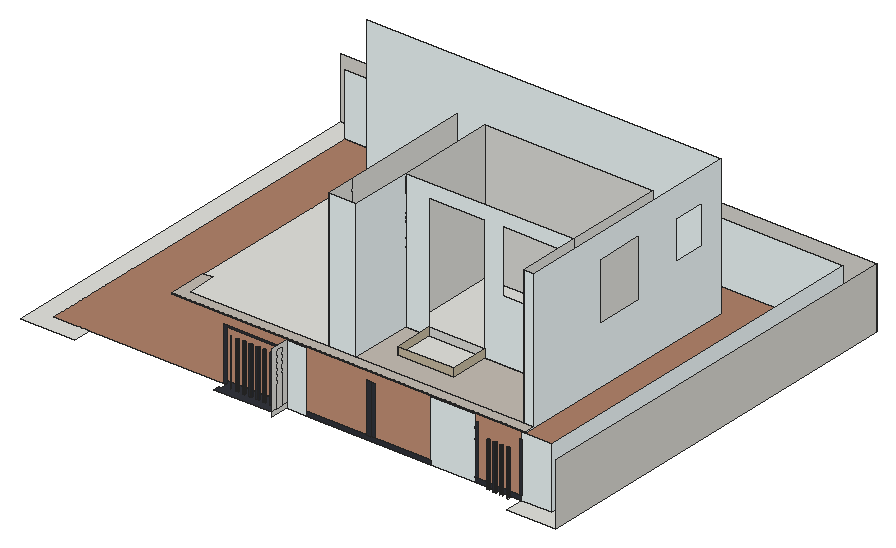
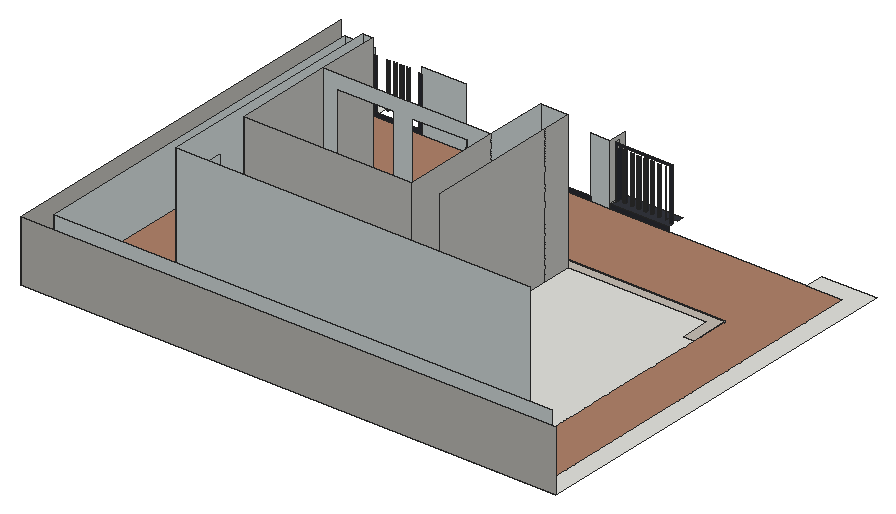
# SketchUp Ruby script. Lengths in inches.
U = 1.inch
M = Sketchup.active_model
def pt(a) = Geom::Point3d.new(a.map { |v| v * U })
def face(e, loops, mat)
  f = e.add_face(loops[0].map { |a| pt(a) })
  loops[1..].each { |l| e.add_face(l.map { |a| pt(a) }).erase! }
  f.material = f.back_material = mat if mat
  f
end
# faces: each face lists its corners as indices into pts; further lists are holes
def faces(e, pts, list, mat = nil) = list.each { |f| face(e, (f[0].is_a?(Array) ? f : [f]).map { |l| l.map { |i| pts[i] } }, mat) }
# xy, xz, yz: faces in a plane at the given z, y or x. An outline is a flat list of corners, or four numbers for a rectangle; further outlines are holes
def ring(l) = l.size == 4 ? [[l[0], l[1]], [l[2], l[1]], [l[2], l[3]], [l[0], l[3]]] : l.each_slice(2).to_a
def flat(e, list, mat, &to3) = list.each { |f| face(e, (f[0].is_a?(Array) ? f : [f]).map { |l| ring(l).map { |u, v| to3.(u, v) } }, mat) }
def xy(e, z, list, mat = nil) = flat(e, list, mat) { |x, y| [x, y, z] }
def xz(e, y, list, mat = nil) = flat(e, list, mat) { |x, z| [x, y, z] }
def yz(e, x, list, mat = nil) = flat(e, list, mat) { |y, z| [x, y, z] }
def lines(e, pts, list) = list.each { |a, b| e.add_line(pt(pts[a]), pt(pts[b])) }
# prism: a flat outline (further loops are holes) pulled along v
def prism(e, loops, v, mat = nil)
  f = face(e, loops, mat); d = Geom::Vector3d.new(v.map { |x| x * U })
  f.pushpull(f.normal.samedirection?(d) ? d.length : -d.length)
end
def box(e, o, s, mat = nil) = prism(e, [[o, [o[0] + s[0], o[1], o[2]], [o[0] + s[0], o[1] + s[1], o[2]], [o[0], o[1] + s[1], o[2]]]], [0, 0, s[2]], mat)
def at(x, y, z, deg = 0) = Geom::Transformation.translation(pt([x, y, z])) * Geom::Transformation.rotation(ORIGIN, Z_AXIS, deg.degrees)
def axes(o, x, y, z) = Geom::Transformation.new([*x, 0, *y, 0, *z, 0, *pt(o).to_a, 1])
def part(name) = M.definitions.add(name)
# library, detail: a bought-in or finely detailed component or shape, given as its bounding box
def library(name, o, s) = part(name).tap { |d| box(d.entities, o, s) }
def detail(e, o, s) = box(e.add_group.entities, o, s)
def put(e, d, t, mat = nil) = e.add_instance(d, t).tap { |i| i.material = mat if mat }
def group(e, t, mat = nil) = e.add_group.tap { |g| g.transformation = t; g.material = mat if mat }.entities
root = M.entities
M.materials.add("[Concrete Tile]").color = [203, 190, 164]
M.materials.add("[Field Rectangle Tile]").color = [196, 189, 179]
M.materials.add("[Formica Laminate Dark]1").color = [50, 53, 60]
M.materials.add("[Pavers Driveway Brick]").color = [176, 130, 106]
M.materials.add("[Terrazzo Tile Light]").color = [219, 217, 210]
M.materials.add("[White Subway Tile]").color = [243, 252, 253]
M.materials.add("[White Subway Tile]1").color = [243, 252, 253]
xy(root,0,[[0,0,0,2816.0625,3762.625,2816.0625,3762.625,0,3421.78,0,3421.78,129.42,3633.2,129.42,3633.2,2686.64,129.42,2686.64,129.42,129.42,383.65,129.42,383.65,0],[477.43,733.79,2968.68,2442.87]])
xy(root,0,[[[129.42,129.42,3633.2,2686.64],[477.43,733.79,2968.68,2442.87]]],"[Pavers Driveway Brick]")
xy(root,9,[[1882.4375,963.83,2273.5625,1239.01],[1717.43,1239.01,2898.76,1933.89]])
xy(root,9,[[477.43,733.79,2968.68,733.79,2968.68,803.71,547.35,803.71,547.35,1008.89,477.43,1008.89],[1717.43,803.71,2898.76,803.71,2898.76,1239.01,2273.5625,1239.01,2273.5625,963.83,1882.4375,963.83,1882.4375,1239.01,1717.43,1239.01]],"[Field Rectangle Tile]")
xy(root,29.875,[[3376.3,55.58,3373.8,55.72,3371.41,56.51,3369.31,57.89,3367.64,59.76,3366.51,62.01,3365.99,64.47,3366.14,66.98,3366.92,69.36,3368.3,71.46,3370.18,73.14,3372.42,74.27,3374.88,74.78,3377.39,74.64,3379.77,73.85,3381.875,72.47,3383.55,70.6,3384.68,68.35,3385.19,65.89,3385.05,63.38,3384.26,61,3382.88,58.9,3381.01,57.22,3378.76,56.09]])
xy(root,29.875,[[[1357.59,0,1765.91,0,1765.91,44.85,1752.89,44.85,1752.89,92.78,1765.91,92.78,1765.91,129.42,1357.59,129.42,1357.59,92.78,1376.86,92.78,1376.86,44.85,1357.59,44.85],[1663.87,55.58,1661.36,55.72,1658.97,56.51,1656.87,57.89,1655.2,59.76,1654.07,62.01,1653.56,64.47,1653.7,66.98,1654.49,69.36,1655.86,71.46,1657.74,73.14,1659.98,74.27,1662.44,74.78,1664.95,74.64,1667.34,73.85,1669.4375,72.47,1671.11,70.6,1672.24,68.35,1672.75,65.89,1672.61,63.38,1671.82,61,1670.45,58.9,1668.57,57.22,1666.33,56.09],[1417.24,55.58,1414.73,55.72,1412.35,56.51,1410.25,57.89,1408.57,59.76,1407.44,62.01,1406.93,64.47,1407.07,66.98,1407.86,69.36,1409.24,71.46,1411.11,73.14,1413.36,74.27,1415.82,74.78,1418.33,74.64,1420.71,73.85,1422.8125,72.47,1424.49,70.6,1425.62,68.35,1426.13,65.89,1425.99,63.38,1425.2,61,1423.82,58.9,1421.95,57.22,1419.7,56.09],[1616.43,55.58,1613.92,55.72,1611.54,56.51,1609.43,57.89,1607.76,59.76,1606.63,62.01,1606.12,64.47,1606.26,66.98,1607.05,69.36,1608.43,71.46,1610.3,73.14,1612.54,74.27,1615,74.78,1617.51,74.64,1619.9,73.85,1622,72.47,1623.67,70.6,1624.8,68.35,1625.32,65.89,1625.17,63.38,1624.39,61,1623.01,58.9,1621.13,57.22,1618.89,56.09],[1472.87,55.58,1470.36,55.72,1467.97,56.51,1465.87,57.89,1464.2,59.76,1463.07,62.01,1462.56,64.47,1462.7,66.98,1463.49,69.36,1464.86,71.46,1466.74,73.14,1468.98,74.27,1471.44,74.78,1473.95,74.64,1476.34,73.85,1478.4375,72.47,1480.11,70.6,1481.24,68.35,1481.75,65.89,1481.61,63.38,1480.82,61,1479.45,58.9,1477.57,57.22,1475.33,56.09],[1518.99,55.58,1516.48,55.72,1514.1,56.51,1512,57.89,1510.32,59.76,1509.19,62.01,1508.68,64.47,1508.82,66.98,1509.61,69.36,1510.99,71.46,1512.86,73.14,1515.11,74.27,1517.57,74.78,1520.08,74.64,1522.46,73.85,1524.5625,72.47,1526.24,70.6,1527.37,68.35,1527.88,65.89,1527.74,63.38,1526.95,61,1525.57,58.9,1523.7,57.22,1521.45,56.09],[1714.37,55.58,1711.86,55.72,1709.47,56.51,1707.37,57.89,1705.7,59.76,1704.57,62.01,1704.06,64.47,1704.2,66.98,1704.99,69.36,1706.36,71.46,1708.24,73.14,1710.48,74.27,1712.94,74.78,1715.45,74.64,1717.84,73.85,1719.9375,72.47,1721.61,70.6,1722.74,68.35,1723.25,65.89,1723.11,63.38,1722.32,61,1720.95,58.9,1719.07,57.22,1716.83,56.09],[1566.87,55.58,1564.36,55.72,1561.97,56.51,1559.87,57.89,1558.2,59.76,1557.07,62.01,1556.56,64.47,1556.7,66.98,1557.49,69.36,1558.86,71.46,1560.74,73.14,1562.98,74.27,1565.44,74.78,1567.95,74.64,1570.34,73.85,1572.4375,72.47,1574.11,70.6,1575.24,68.35,1575.75,65.89,1575.61,63.38,1574.82,61,1573.45,58.9,1571.57,57.22,1569.33,56.09]]],"[Formica Laminate Dark]1")
xz(root,92.78,[[1357.59,29.875,1357.59,402.23,1765.91,402.23,1765.91,29.875,1752.89,29.875,1752.89,387.92,1376.86,387.92,1376.86,29.875]],"[Formica Laminate Dark]1")
xz(root,129.42,[[1357.59,0,1765.91,29.875],[1905.75,0,2778.47,29.875],[3092.67,0,3421.78,29.875],[2330.84,29.875,2358.7,373.47],[2358.7,29.875,2386.55,373.47],
  [3092.67,29.875,3111.49,384.04],[3407.39,29.875,3421.78,384.04]],"[Formica Laminate Dark]1")
xz(root,129.42,[[1765.91,0,1905.75,429.3125],[2778.47,0,3092.67,429.3125],[3421.78,0,3633.2,429.3125]],"[White Subway Tile]1")
xz(root,733.79,[[477.43,0,2968.68,9]])
xz(root,803.71,[[1522.59,9,1717.43,973.375],[2898.76,9,2968.68,973.375]],"[White Subway Tile]")
xz(root,963.83,[[1882.4375,9,2273.5625,62.21]],"[Concrete Tile]")
xz(root,1239.01,[[1882.4375,9,2273.5625,62.21]])
xz(root,1239.01,[[[1717.43,9,1882.4375,9,1882.4375,877.21,2273.5625,877.21,2273.5625,9,2898.76,9,2898.76,973.375,1717.43,973.375],[2398.08,439.46,2800.45,879.09]]],"[White Subway Tile]")
xz(root,1933.89,[[1717.43,9,2898.76,973.375]])
xz(root,2442.87,[[477.43,0,2968.68,973.375]],"[White Subway Tile]")
xz(root,2686.64,[[129.42,0,3633.2,429.3125]],"[White Subway Tile]1")
xz(root,2816.0625,[[0,0,3762.625,429.3125]],"[Terrazzo Tile Light]")
yz(root,1522.59,[[803.71,9,1008.89,973.375],[1008.89,9,1933.89,973.375]])
yz(root,1717.43,[[1239.01,9,1933.89,973.375]])
yz(root,1717.43,[[803.71,9,1239.01,973.375]],"[White Subway Tile]")
yz(root,1752.89,[[44.85,29.875,92.78,357.02]],"[Formica Laminate Dark]1")
yz(root,1765.91,[[0,0,129.42,29.875],[0,29.875,0,429.3125,129.42,429.3125,129.42,29.875,92.78,29.875,92.78,402.23,44.85,402.23,44.85,29.875],[44.85,29.875,92.78,402.23]])
yz(root,1882.4375,[[963.83,9,1239.01,62.21]],"[Concrete Tile]")
yz(root,2273.5625,[[963.83,9,1239.01,62.21]],"[Concrete Tile]")
yz(root,2898.76,[[803.71,9,1239.01,973.375],[1239.01,9,1933.89,973.375]])
yz(root,2968.68,[[[733.79,0,2442.87,0,2442.87,973.375,803.71,973.375,803.71,9,733.79,9],[1375.57,402.84,1724.7,809.34],[2046.63,498.46,2278.38,771.33]]],"[White Subway Tile]")
yz(root,3633.2,[[129.42,0,2686.64,429.3125]],"[White Subway Tile]1")
yz(root,3762.625,[[0,0,2816.0625,429.3125]],"[Terrazzo Tile Light]")
p = [[1462.7,66.98,29.875],[1462.56,64.47,29.875],[1462.56,64.47,357.02],[1462.7,66.98,357.02],[1508.82,66.98,29.875],[1508.68,64.47,29.875],
  [1508.68,64.47,357.02],[1508.82,66.98,357.02],[1556.7,66.98,29.875],[1556.56,64.47,29.875],[1556.56,64.47,357.02],[1556.7,66.98,357.02],
  [1606.26,66.98,29.875],[1606.12,64.47,29.875],[1606.12,64.47,357.02],[1606.26,66.98,357.02],[1653.7,66.98,29.875],[1653.56,64.47,29.875],
  [1653.56,64.47,357.02],[1653.7,66.98,357.02],[1704.2,66.98,29.875],[1704.06,64.47,29.875],[1704.06,64.47,357.02],[1704.2,66.98,357.02],
  [3226.76,66.98,29.875],[3226.62,64.47,29.875],[3226.62,64.47,342.54],[3226.76,66.98,342.54],[3272.39,66.98,29.875],[3272.24,64.47,29.875],
  [3272.24,64.47,342.54],[3272.39,66.98,342.54],[3318.51,66.98,29.875],[3318.37,64.47,29.875],[3318.37,64.47,342.54],[3318.51,66.98,342.54],
  [3366.14,66.98,29.875],[3365.99,64.47,29.875],[3365.99,64.47,342.54],[3366.14,66.98,342.54],[1426.13,65.89,29.875],[1425.62,68.35,29.875],
  [1425.62,68.35,357.02],[1426.13,65.89,357.02],[1481.75,65.89,29.875],[1481.24,68.35,29.875],[1481.24,68.35,357.02],[1481.75,65.89,357.02],
  [1527.88,65.89,29.875],[1527.37,68.35,29.875],[1527.37,68.35,357.02],[1527.88,65.89,357.02],[1575.75,65.89,29.875],[1575.24,68.35,29.875],
  [1575.24,68.35,357.02],[1575.75,65.89,357.02],[1625.32,65.89,29.875],[1624.8,68.35,29.875],[1624.8,68.35,357.02],[1625.32,65.89,357.02],
  [1672.75,65.89,29.875],[1672.24,68.35,29.875],[1672.24,68.35,357.02],[1672.75,65.89,357.02],[1723.25,65.89,29.875],[1722.74,68.35,29.875],
  [1722.74,68.35,357.02],[1723.25,65.89,357.02],[3245.82,65.89,29.875],[3245.3,68.35,29.875],[3245.3,68.35,342.54],[3245.82,65.89,342.54],
  [3291.44,65.89,29.875],[3290.93,68.35,29.875],[3290.93,68.35,342.54],[3291.44,65.89,342.54],[3337.57,65.89,29.875],[3337.05,68.35,29.875],
  [3337.05,68.35,342.54],[3337.57,65.89,342.54],[3385.19,65.89,29.875],[3384.68,68.35,29.875],[3384.68,68.35,342.54],[3385.19,65.89,342.54],
  [1463.49,69.36,29.875],[1463.49,69.36,357.02],[1509.61,69.36,29.875],[1509.61,69.36,357.02],[1557.49,69.36,29.875],[1557.49,69.36,357.02],
  [1607.05,69.36,29.875],[1607.05,69.36,357.02],[1654.49,69.36,29.875],[1654.49,69.36,357.02],[1704.99,69.36,29.875],[1704.99,69.36,357.02],
  [3227.55,69.36,29.875],[3227.55,69.36,342.54],[3273.17,69.36,29.875],[3273.17,69.36,342.54],[3319.3,69.36,29.875],[3319.3,69.36,342.54],
  [3366.92,69.36,29.875],[3366.92,69.36,342.54],[1424.49,70.6,29.875],[1424.49,70.6,357.02],[1480.11,70.6,29.875],[1480.11,70.6,357.02],
  [1526.24,70.6,29.875],[1526.24,70.6,357.02],[1574.11,70.6,29.875],[1574.11,70.6,357.02],[1623.67,70.6,29.875],[1623.67,70.6,357.02],
  [1671.11,70.6,29.875],[1671.11,70.6,357.02],[1721.61,70.6,29.875],[1721.61,70.6,357.02],[3244.17,70.6,29.875],[3244.17,70.6,342.54],
  [3289.8,70.6,29.875],[3289.8,70.6,342.54],[3335.92,70.6,29.875],[3335.92,70.6,342.54],[3383.55,70.6,29.875],[3383.55,70.6,342.54],
  [1464.86,71.46,29.875],[1464.86,71.46,357.02],[1510.99,71.46,29.875],[1510.99,71.46,357.02],[1558.86,71.46,29.875],[1558.86,71.46,357.02],
  [1608.43,71.46,29.875],[1608.43,71.46,357.02],[1655.86,71.46,29.875],[1655.86,71.46,357.02],[1706.36,71.46,29.875],[1706.36,71.46,357.02],
  [3228.93,71.46,29.875],[3228.93,71.46,342.54],[3274.55,71.46,29.875],[3274.55,71.46,342.54],[3320.68,71.46,29.875],[3320.68,71.46,342.54],
  [3368.3,71.46,29.875],[3368.3,71.46,342.54],[1422.8125,72.47,29.875],[1422.8125,72.47,357.02],[1478.4375,72.47,29.875],[1478.4375,72.47,357.02],
  [1524.5625,72.47,29.875],[1524.5625,72.47,357.02],[1572.4375,72.47,29.875],[1572.4375,72.47,357.02],[1622,72.47,29.875],[1622,72.47,357.02],
  [1669.4375,72.47,29.875],[1669.4375,72.47,357.02],[1719.9375,72.47,29.875],[1719.9375,72.47,357.02],[3242.5,72.47,29.875],[3242.5,72.47,342.54],
  [3288.125,72.47,29.875],[3288.125,72.47,342.54],[3334.25,72.47,29.875],[3334.25,72.47,342.54],[3381.875,72.47,29.875],[3381.875,72.47,342.54],
  [1466.74,73.14,29.875],[1466.74,73.14,357.02],[1512.86,73.14,29.875],[1512.86,73.14,357.02],[1560.74,73.14,29.875],[1560.74,73.14,357.02],
  [1610.3,73.14,29.875],[1610.3,73.14,357.02],[1657.74,73.14,29.875],[1657.74,73.14,357.02],[1708.24,73.14,29.875],[1708.24,73.14,357.02],
  [3230.8,73.14,29.875],[3230.8,73.14,342.54],[3276.43,73.14,29.875],[3276.43,73.14,342.54],[3322.55,73.14,29.875],[3322.55,73.14,342.54],
  [3370.18,73.14,29.875],[3370.18,73.14,342.54],[1420.71,73.85,29.875],[1420.71,73.85,357.02],[1476.34,73.85,29.875],[1476.34,73.85,357.02],
  [1522.46,73.85,29.875],[1522.46,73.85,357.02],[1570.34,73.85,29.875],[1570.34,73.85,357.02],[1619.9,73.85,29.875],[1619.9,73.85,357.02],
  [1667.34,73.85,29.875],[1667.34,73.85,357.02],[1717.84,73.85,29.875],[1717.84,73.85,357.02],[3240.4,73.85,29.875],[3240.4,73.85,342.54],
  [3286.02,73.85,29.875],[3286.02,73.85,342.54],[3332.15,73.85,29.875],[3332.15,73.85,342.54],[3379.77,73.85,29.875],[3379.77,73.85,342.54],
  [1468.98,74.27,29.875],[1468.98,74.27,357.02],[1515.11,74.27,29.875],[1515.11,74.27,357.02],[1562.98,74.27,29.875],[1562.98,74.27,357.02],
  [1612.54,74.27,29.875],[1612.54,74.27,357.02],[1659.98,74.27,29.875],[1659.98,74.27,357.02],[1710.48,74.27,29.875],[1710.48,74.27,357.02],
  [3233.04,74.27,29.875],[3233.04,74.27,342.54],[3278.67,74.27,29.875],[3278.67,74.27,342.54],[3324.79,74.27,29.875],[3324.79,74.27,342.54],
  [3372.42,74.27,29.875],[3372.42,74.27,342.54],[1418.33,74.64,29.875],[1418.33,74.64,357.02],[1473.95,74.64,29.875],[1473.95,74.64,357.02],
  [1520.08,74.64,29.875],[1520.08,74.64,357.02],[1567.95,74.64,29.875],[1567.95,74.64,357.02],[1617.51,74.64,29.875],[1617.51,74.64,357.02],
  [1664.95,74.64,29.875],[1664.95,74.64,357.02],[1715.45,74.64,29.875],[1715.45,74.64,357.02],[3238.01,74.64,29.875],[3238.01,74.64,342.54],
  [3283.64,74.64,29.875],[3283.64,74.64,342.54],[3329.76,74.64,29.875],[3329.76,74.64,342.54],[3377.39,74.64,29.875],[3377.39,74.64,342.54],
  [1471.44,74.78,29.875],[1471.44,74.78,357.02],[1517.57,74.78,29.875],[1517.57,74.78,357.02],[1565.44,74.78,29.875],[1565.44,74.78,357.02],
  [1615,74.78,29.875],[1615,74.78,357.02],[1662.44,74.78,29.875],[1662.44,74.78,357.02],[1712.94,74.78,29.875],[1712.94,74.78,357.02],
  [3235.5,74.78,29.875],[3235.5,74.78,342.54],[3281.13,74.78,29.875],[3281.13,74.78,342.54],[3327.25,74.78,29.875],[3327.25,74.78,342.54],
  [3374.88,74.78,29.875],[3374.88,74.78,342.54]]
faces(root,p,[[0,1,2,3],[4,5,6,7],[8,9,10,11],[12,13,14,15],[16,17,18,19],[20,21,22,23],[24,25,26,27],[28,29,30,31],
  [32,33,34,35],[36,37,38,39],[40,41,42,43],[44,45,46,47],[48,49,50,51],[52,53,54,55],[56,57,58,59],[60,61,62,63],
  [64,65,66,67],[68,69,70,71],[72,73,74,75],[76,77,78,79],[80,81,82,83],[84,0,3,85],[86,4,7,87],[88,8,11,89],
  [90,12,15,91],[92,16,19,93],[94,20,23,95],[96,24,27,97],[98,28,31,99],[100,32,35,101],[102,36,39,103],[41,104,105,42],
  [45,106,107,46],[49,108,109,50],[53,110,111,54],[57,112,113,58],[61,114,115,62],[65,116,117,66],[69,118,119,70],[73,120,121,74],
  [77,122,123,78],[81,124,125,82],[126,84,85,127],[128,86,87,129],[130,88,89,131],[132,90,91,133],[134,92,93,135],[136,94,95,137],
  [138,96,97,139],[140,98,99,141],[142,100,101,143],[144,102,103,145],[104,146,147,105],[106,148,149,107],[108,150,151,109],[110,152,153,111],
  [112,154,155,113],[114,156,157,115],[116,158,159,117],[118,160,161,119],[120,162,163,121],[122,164,165,123],[124,166,167,125],[168,126,127,169],
  [170,128,129,171],[172,130,131,173],[174,132,133,175],[176,134,135,177],[178,136,137,179],[180,138,139,181],[182,140,141,183],[184,142,143,185],
  [186,144,145,187],[146,188,189,147],[148,190,191,149],[150,192,193,151],[152,194,195,153],[154,196,197,155],[156,198,199,157],[158,200,201,159],
  [160,202,203,161],[162,204,205,163],[164,206,207,165],[166,208,209,167],[210,168,169,211],[212,170,171,213],[214,172,173,215],[216,174,175,217],
  [218,176,177,219],[220,178,179,221],[222,180,181,223],[224,182,183,225],[226,184,185,227],[228,186,187,229],[188,230,231,189],[190,232,233,191],
  [192,234,235,193],[194,236,237,195],[196,238,239,197],[198,240,241,199],[200,242,243,201],[202,244,245,203],[204,246,247,205],[206,248,249,207],
  [208,250,251,209],[252,210,211,253],[254,212,213,255],[256,214,215,257],[258,216,217,259],[260,218,219,261],[262,220,221,263],[264,222,223,265],
  [266,224,225,267],[268,226,227,269],[270,228,229,271],[232,252,253,233],[234,254,255,235],[236,256,257,237],[238,258,259,239],[240,260,261,241],
  [242,262,263,243],[244,264,265,245],[246,266,267,247],[248,268,269,249],[250,270,271,251]],"[Formica Laminate Dark]1")
